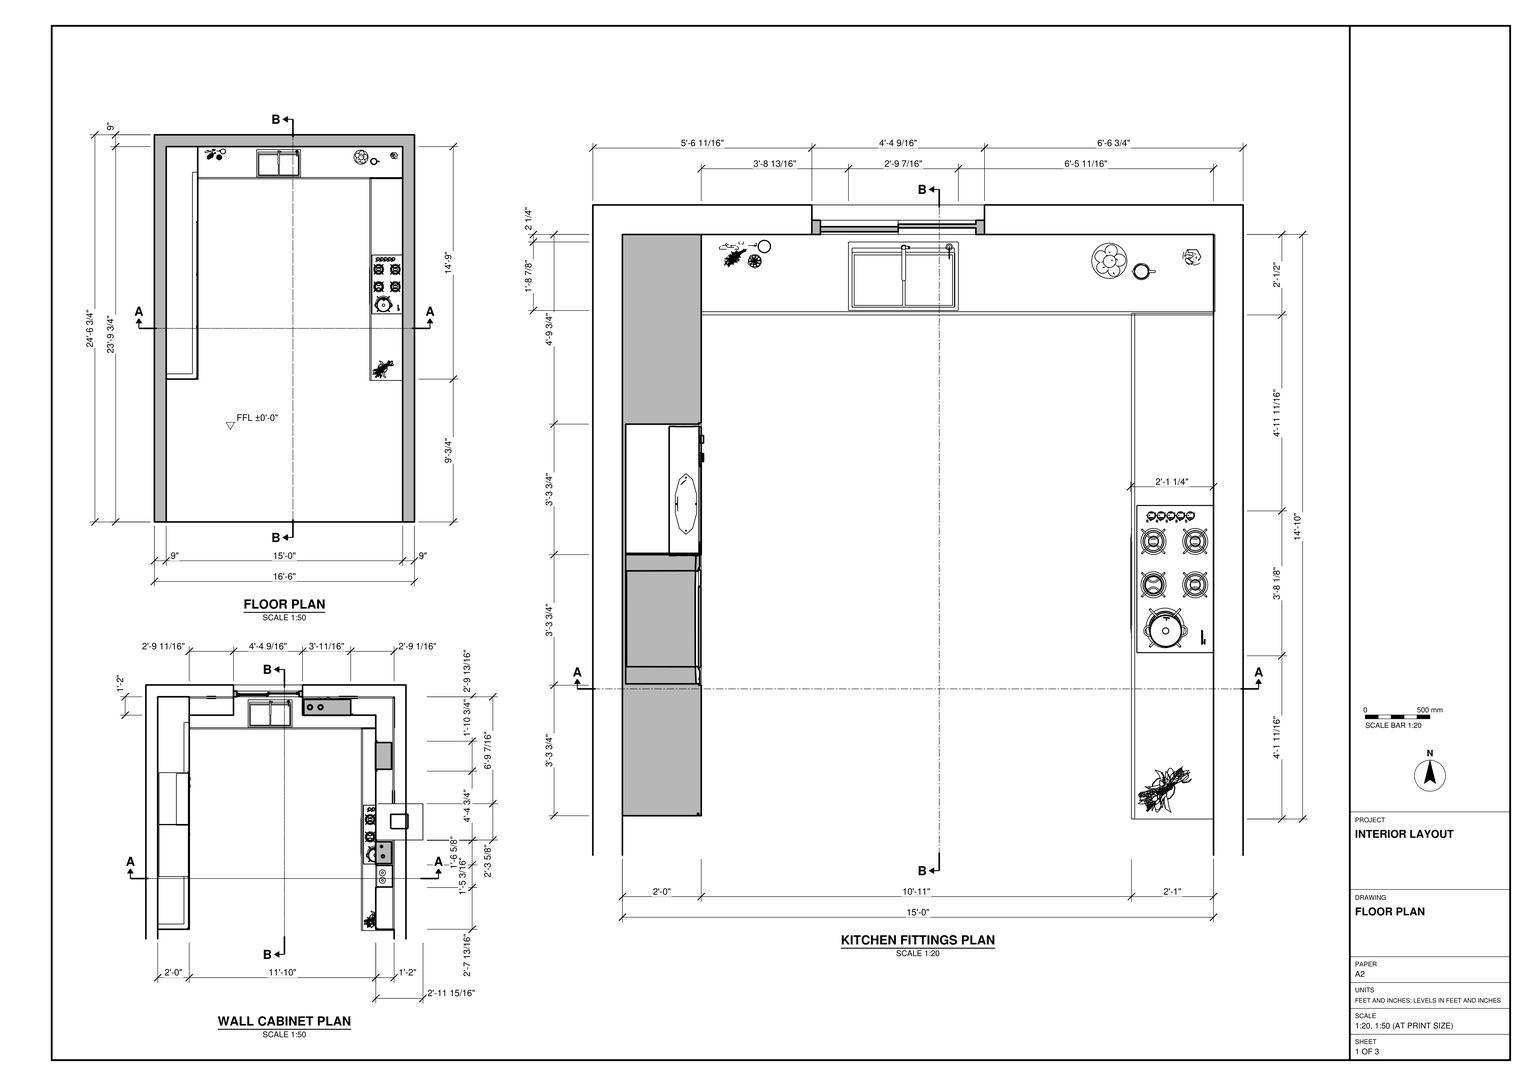
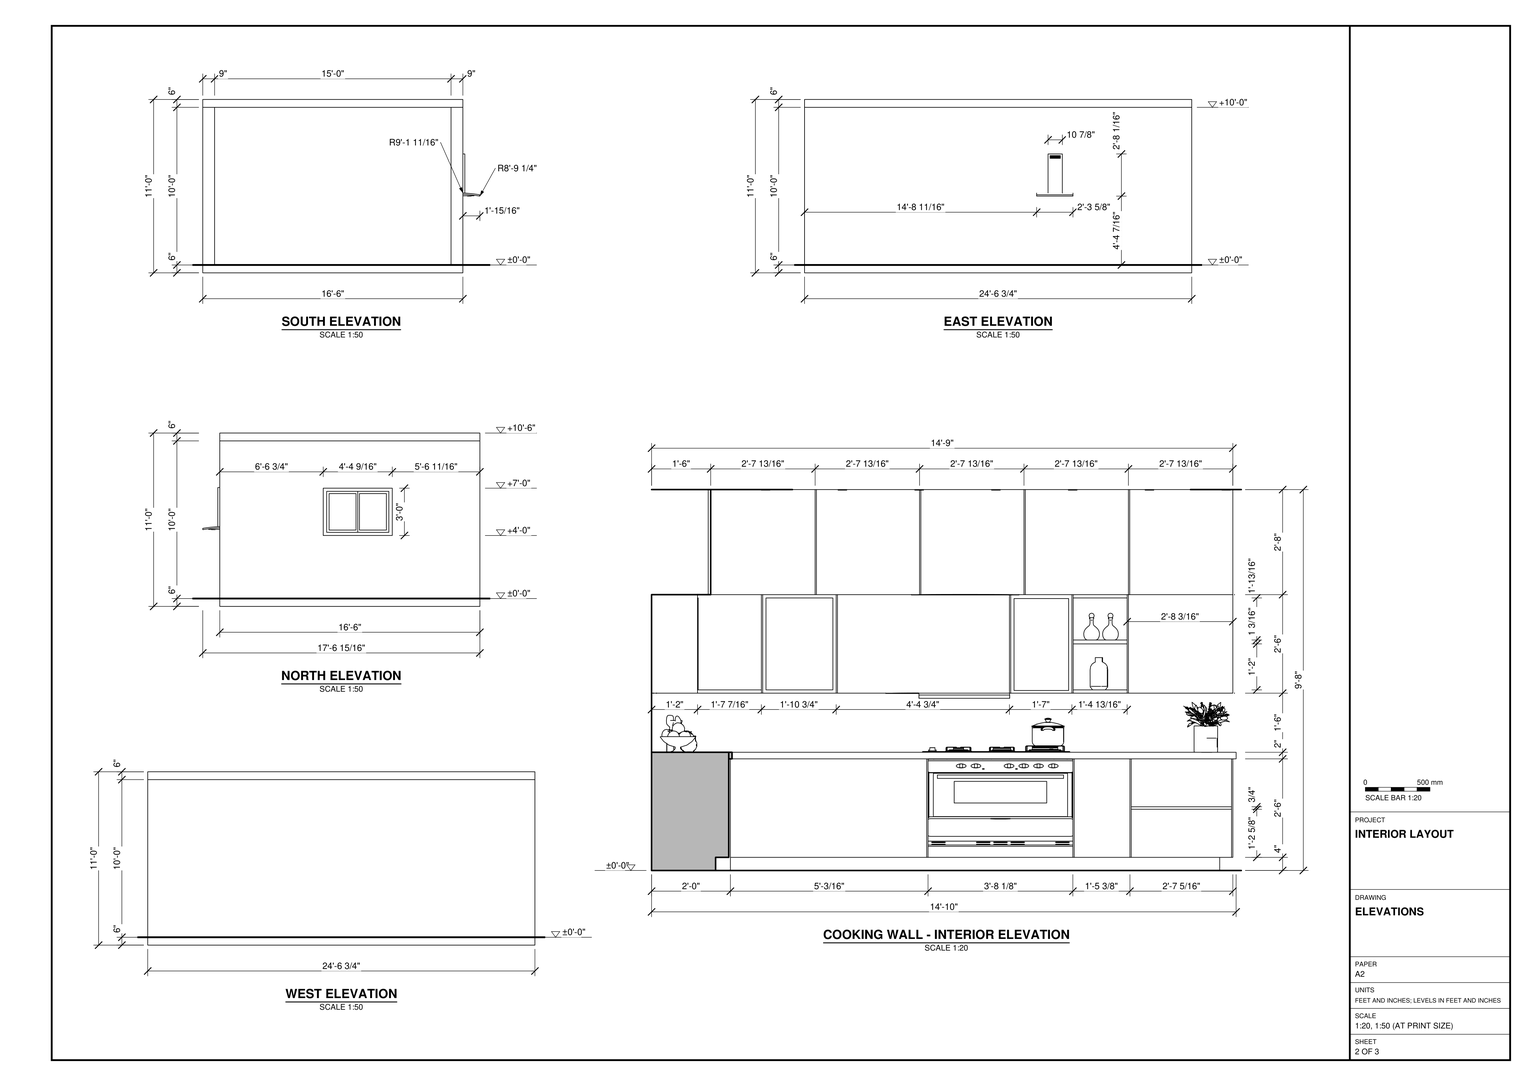
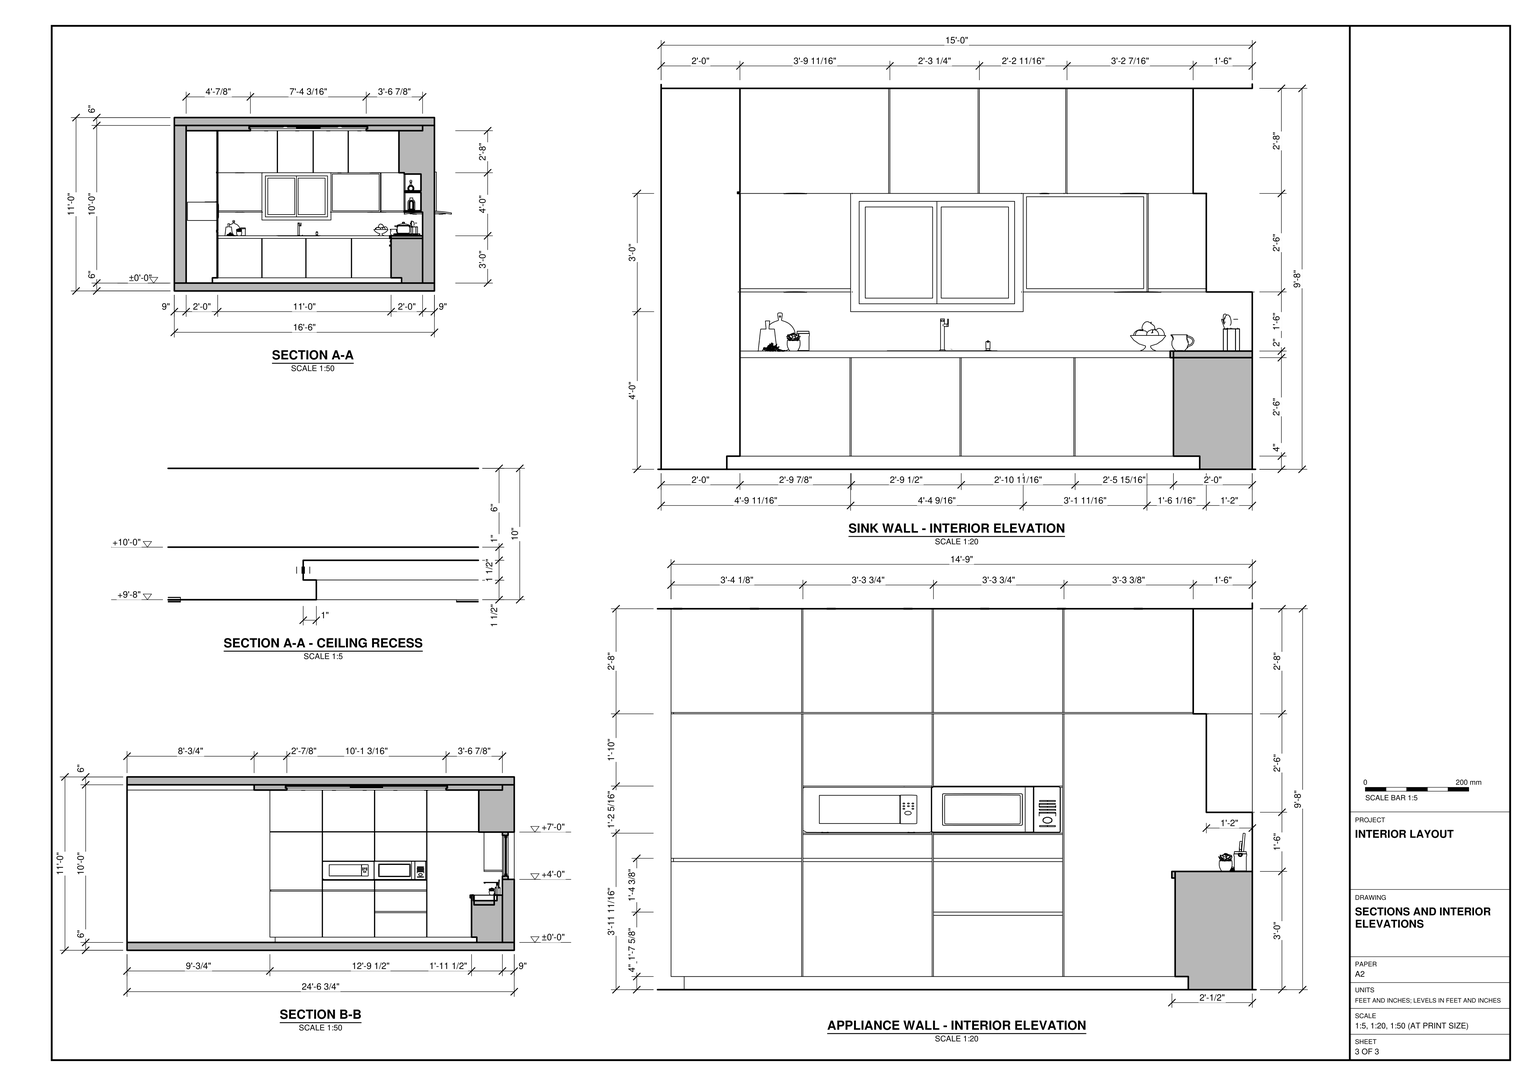
Build the kitchen interior in SketchUp from task_files/diagram_01.pdf. Work in feet and inches, with the finished floor at ±0'-0". The overall model extents, including the projection at the cooking wall, are 17'-6 15/16" wide, 24'-6 3/4" deep and 11'-0" high. Keep the room itself 15'-0" wide between the inside faces of the side walls. Model the 9" walls, the open south end, the floor and ceiling slabs, and the stepped ceiling recess shown in section.

Use the fittings plan to lay out the three cabinet runs and the interior elevations to divide their fronts. On the north wall, place the double-bowl sink and tap beneath the two-panel window, with base cupboards below the counter and wall cabinets around the opening. On the east wall, align the cooktop, oven and hood, and include the open shelf bay beside the hood. On the opposite wall, fit the two appliances side by side within the tall cabinetry. Leave the aisle and the floor toward the open end clear. Appliances, plants and loose countertop items may be any suitable library components placed as shown.

Keep the shell elements and each joinery piece in separate groups or components, and use components for repeated parts. Save one SketchUp model as output_files/u_shaped_kitchen_with_fitted_cabinetry.skp.

# SketchUp Ruby script. Lengths in inches.
U = 1.inch
M = Sketchup.active_model
def pt(a) = Geom::Point3d.new(a.map { |v| v * U })
def face(e, loops, mat)
  f = e.add_face(loops[0].map { |a| pt(a) })
  loops[1..].each { |l| e.add_face(l.map { |a| pt(a) }).erase! }
  f.material = f.back_material = mat if mat
  f
end
# faces: each face lists its corners as indices into pts; further lists are holes
def faces(e, pts, list, mat = nil) = list.each { |f| face(e, (f[0].is_a?(Array) ? f : [f]).map { |l| l.map { |i| pts[i] } }, mat) }
# xy, xz, yz: faces in a plane at the given z, y or x. An outline is a flat list of corners, or four numbers for a rectangle; further outlines are holes
def ring(l) = l.size == 4 ? [[l[0], l[1]], [l[2], l[1]], [l[2], l[3]], [l[0], l[3]]] : l.each_slice(2).to_a
def flat(e, list, mat, &to3) = list.each { |f| face(e, (f[0].is_a?(Array) ? f : [f]).map { |l| ring(l).map { |u, v| to3.(u, v) } }, mat) }
def xy(e, z, list, mat = nil) = flat(e, list, mat) { |x, y| [x, y, z] }
def xz(e, y, list, mat = nil) = flat(e, list, mat) { |x, z| [x, y, z] }
def yz(e, x, list, mat = nil) = flat(e, list, mat) { |y, z| [x, y, z] }
def lines(e, pts, list) = list.each { |a, b| e.add_line(pt(pts[a]), pt(pts[b])) }
# prism: a flat outline (further loops are holes) pulled along v
def prism(e, loops, v, mat = nil)
  f = face(e, loops, mat); d = Geom::Vector3d.new(v.map { |x| x * U })
  f.pushpull(f.normal.samedirection?(d) ? d.length : -d.length)
end
def box(e, o, s, mat = nil) = prism(e, [[o, [o[0] + s[0], o[1], o[2]], [o[0] + s[0], o[1] + s[1], o[2]], [o[0], o[1] + s[1], o[2]]]], [0, 0, s[2]], mat)
def at(x, y, z, deg = 0) = Geom::Transformation.translation(pt([x, y, z])) * Geom::Transformation.rotation(ORIGIN, Z_AXIS, deg.degrees)
def axes(o, x, y, z) = Geom::Transformation.new([*x, 0, *y, 0, *z, 0, *pt(o).to_a, 1])
def part(name) = M.definitions.add(name)
# library, detail: a bought-in or finely detailed component or shape, given as its bounding box
def library(name, o, s) = part(name).tap { |d| box(d.entities, o, s) }
def detail(e, o, s) = box(e.add_group.entities, o, s)
def put(e, d, t, mat = nil) = e.add_instance(d, t).tap { |i| i.material = mat if mat }
def group(e, t, mat = nil) = e.add_group.tap { |g| g.transformation = t; g.material = mat if mat }.entities
root = M.entities
M.materials.add("0209 AP 9428 SKY PINK").color = [243, 236, 233]
M.materials.add("Emissive").color = [244, 243, 201]
M.materials.add("Generic").color = [193, 202, 184]
M.materials.add("Glass Thin Clear 001\#1").color = [29, 27, 27]
M.materials["Glass Thin Clear 001\#1"].alpha = 0.1
M.materials.add("Granite Black Pearl 150cm").color = [48, 48, 48]
M.materials.add("Tiles Simple 02 100cm\#1").color = [183, 183, 183]
M.materials.add("[Color M08]").color = [30, 30, 30]
M.materials.add("[Translucent_Glass_Safety]").color = [204, 235, 244]
M.materials["[Translucent_Glass_Safety]"].alpha = 0.5
M.materials.add("[Translucent_Glass_Sky_Reflection]").color = [125, 138, 183]
M.materials["[Translucent_Glass_Sky_Reflection]"].alpha = 0.52
M.materials.add("[Wood Floor Light]").color = [204, 176, 127]
c1 = library("Microwave 116-15",[-11.91,-6.3,0],[23.82,12.61,15.33])
c2 = library("Microwave 116-11",[-7.27,-5.23,0],[14.54,10.46,7.87])
c3 = library("Utensils",[0,-0.54,-0.24],[6.34,6.28,13.37])
c4 = library("Glass_Apothecary_Jar",[-11.5,-3.52,0],[30.82,7.02,10])
c5 = library("ACCESS \#103",[-1.07,0,-1.17],[14.88,24.44,20.18])
c6 = library("Kitchen Utensils - Pot",[14.77,-5.37,0.11],[13.29,9.84,8.54])
c7 = library("kitchen utensils1",[32.53,200.33,5.92],[41.29,12.2,17.07])
c8 = part("Sliding window")
xy(c8.entities,0,[[0,0,4.33,55.51]])
xy(c8.entities,2.76,[[0,2.76,2,27.76],[3.15,2.76,4.33,27.76],[0,27.76,0.82,52.76],[0.82,27.76,2.36,52.76],[2.36,27.76,4.33,52.76]])
xy(c8.entities,4.72,[[2,4.72,2.4,26.38],[2.76,4.72,3.15,26.38],[0.82,29.13,1.22,50.79],[1.97,29.13,2.36,50.79]])
xy(c8.entities,36.61,[[2,4.72,2.4,26.38],[2.76,4.72,3.15,26.38],[0.82,29.13,1.22,50.79],[1.97,29.13,2.36,50.79]])
xy(c8.entities,38.58,[[0,2.76,2,27.76],[3.15,2.76,4.33,27.76],[0,27.76,0.82,52.76],[0.82,27.76,2.36,52.76],[2.36,27.76,4.33,52.76]])
xy(c8.entities,41.34,[[0,0,4.33,55.51]])
xz(c8.entities,0,[[0,0,4.33,41.34]])
xz(c8.entities,2.76,[[0,2.76,2,38.58],[3.15,2.76,4.33,38.58]])
xz(c8.entities,4.72,[[2,4.72,2.4,36.61],[2.76,4.72,3.15,36.61]])
xz(c8.entities,26.38,[[2,4.72,2.4,36.61],[2.76,4.72,3.15,36.61]])
xz(c8.entities,27.76,[[0.82,2.76,2,38.58],[2,2.76,2.36,38.58],[2.36,2.76,3.15,38.58]])
xz(c8.entities,29.13,[[0.82,4.72,1.22,36.61],[1.97,4.72,2.36,36.61]])
xz(c8.entities,50.79,[[0.82,4.72,1.22,36.61],[1.97,4.72,2.36,36.61]])
xz(c8.entities,52.76,[[0,2.76,0.82,38.58],[0.82,2.76,2.36,38.58],[2.36,2.76,4.33,38.58]])
xz(c8.entities,55.51,[[0,0,4.33,41.34]])
yz(c8.entities,0,[[[0,0,55.51,41.34],[2.76,2.76,52.76,38.58]]])
yz(c8.entities,0.82,[[[27.76,2.76,52.76,38.58],[29.13,4.72,50.79,36.61]]])
yz(c8.entities,1.22,[[29.13,4.72,50.79,36.61]],"[Translucent_Glass_Sky_Reflection]")
yz(c8.entities,1.97,[[29.13,4.72,50.79,36.61]],"[Translucent_Glass_Sky_Reflection]")
yz(c8.entities,2,[[[2.76,2.76,27.76,38.58],[4.72,4.72,26.38,36.61]]])
yz(c8.entities,2.36,[[[27.76,2.76,52.76,38.58],[29.13,4.72,50.79,36.61]]])
yz(c8.entities,2.4,[[4.72,4.72,26.38,36.61]],"[Translucent_Glass_Safety]")
yz(c8.entities,2.76,[[4.72,4.72,26.38,36.61]],"[Translucent_Glass_Safety]")
yz(c8.entities,3.15,[[[2.76,2.76,27.76,38.58],[4.72,4.72,26.38,36.61]]])
yz(c8.entities,4.33,[[[0,0,55.51,41.34],[2.76,2.76,52.76,38.58]]])
c9 = library("PV977NSS_GEProfile",[-17.9375,-27.5625,-0.25],[35.95,27.64,32.08])
c10 = library("Cooktop+Brastemp+Ative!",[2.49,1.09,0.39],[33.46,18.11,1.98])
c11 = library("PointStove",[0,-0.4,0],[23.23,24.97,35.55])
c12 = library("Apple 73-11",[-5.39,-5.39,0],[10.78,10.78,8.98])
c13 = library("Vase 193 003",[-7.6875,-7.21,0],[16.1875,14.01,15.28])
c14 = library("Jug 155 004",[-2.86,-2.52,0],[7.11,5.04,4.97])
c15 = library("Bathroom Fixture 02 22-64",[-3.05,-2.36,0],[6.1,4.72,3.64])
c16 = library("Bottle 01 97-27",[-2.41,-2.41,0],[4.82,4.82,8.18])
c17 = library("Bottle 03 97-27",[-1.45,-1.45,0],[2.9,2.9,11.4])
c18 = library("Vase 010",[-2.69,-2.69,0.01],[5.38,5.38,9.84])
c19 = library("white sink",[101.38,33.55,27.24],[20.87,33.46,17.21])
c20 = library("Tlon Light 650 Ceiling 152 007",[-12.8,-12.8,-3.78],[25.6,25.6,3.58])
c21 = library("Group\#25",[-0.5,-0.5,-0.1],[2,177,0.2])
c22 = library("Group\#26",[-0.5,-0.5,-0.1],[70.75,2,0.2])
c23 = library("Group\#27",[-0.5,-0.5,-0.1],[34.6875,2,0.2])
c24 = library("Group\#28",[-0.5,-0.5,-0.1],[34.6875,2,0.2])
c25 = library("Group\#30",[-0.5,-0.5,-0.1],[2.75,164,0.2])
c26 = library("Group\#29",[-0.5,-0.5,-0.1],[42.8125,2.75,0.2])
c27 = library("Group\#31",[-0.5,-0.5,-0.1],[13.9375,2,0.2])
c28 = library("Group\#32",[-0.5,-0.5,0],[90.2,1,1.5])
c29 = library("Group\#33",[-0.5,-0.5,0],[1,123.2,1.5])
c30 = library("Group\#34",[-0.5,-0.5,0],[91.2,1,1.5])
c31 = library("Group\#35",[-0.5,-0.5,0],[1,124.2,1.5])
c32 = library("Group\#36",[-0.5,-0.5,-0.1],[4.4375,102.5625,0.2])
c33 = library("Group\#37",[-0.5,-0.5,-0.1],[4.4375,102.5625,0.2])
xy(root,-6,[[0,0,198,294.75]])
xy(root,0,[[0,0,9,0,9,285.75,189.4375,285.75,189.4375,262.25,189,262.25,189,0,198,0,198,294.75,0,294.75],[9,112.75,9,285.75,33,285.75,33,266.25,29,266.25,29,112.75],[173,112.75,189,261.75],[189,262.25,189.4375,285.75],[33,266.25,189,285.75]])
xy(root,0,[[9,0,189,0,189,112.75,173,112.75,173,261.75,189,261.75,189,266.25,29,266.25,29,112.75,9,112.75]],"Tiles Simple 02 100cm\#1")
xy(root,4,[[9,108.75,9,112.75,29,112.75,29,266.25,33,266.25,33,228.4,32.25,228.4,32.25,228,33,228,33,188.65,32.25,188.65,32.25,188.25,33,188.25,33,148.9,32.25,148.9,32.25,148.5,33,148.5,33,108.75,32.25,108.75,32.25,109.5,31.85,109.5,31.85,108.75],[165.75,108.75,165.75,109.15,165,109.15,165,139.6875,165.75,139.6875,165.75,140.09,165,140.09,165,157.0625,165.75,157.0625,165.75,157.46,165,157.46,165,201.5625,165.75,201.5625,165.75,201.96,165,201.96,165,261.75,173,261.75,173,112.75,169,112.75,169,108.75],[169,108.75,189,112.75],[33,262.25,33,266.25,189,266.25,189,262.25,135.0625,262.25,135.0625,263,134.66,263,134.66,262.25,100.375,262.25,100.375,263,99.98,263,99.98,262.25,66.89,262.25,66.89,263,66.49,263,66.49,262.25]])
xy(root,7.75,[[165,157.46,188,201.5625]])
xy(root,18.65,[[165,109.15,165.75,139.6875]],"[Color M08]")
xy(root,19.4,[[165,109.15,165.75,139.6875]],"[Color M08]")
xy(root,22.625,[[32.25,188.65,33,228]],"[Color M08]")
xy(root,23.625,[[32.25,188.65,33,228]],"[Color M08]")
xy(root,31.8125,[[78.93,263.61,110.08,281.61]],"[Color M08]")
xy(root,34,[[165.75,108.75,165.75,109.15,165,109.15,165,139.6875,165.75,139.6875,165.75,140.09,165,140.09,165,157.0625,165.75,157.0625,165.75,157.46,188,157.46,188,201.5625,165.75,201.5625,165.75,201.96,165,201.96,165,261.25,189,261.25,189,108.75],[165,261.25,189,261.75],[66.49,262.25,66.89,263],[99.98,262.25,100.375,263],[134.66,262.25,135.0625,263]])
xy(root,34,[[164,107.75,165,261.25],[165,107.75,189,108.75],[165,108.75,165.75,109.15],[33,261.25,33,262.25,189,262.25,189,261.75,164,261.75,164,261.25],[164,261.25,165,261.75]],"Granite Black Pearl 150cm")
xy(root,34,[[165,139.6875,165.75,140.09],[165,157.0625,165.75,157.46],[165,157.46,188,201.5625],[165,201.5625,165.75,201.96]],"[Color M08]")
xy(root,36,[[164,261.25,165,261.75],[165,261.25,189,261.75]])
xy(root,36,[[164,107.75,165,261.25],[165,107.75,189,261.25],[33,261.25,164,261.25,164,261.75,189,261.75,189,262.25,33,262.25],[[33,262.25,189,285.75],[78.93,263.61,110.08,281.61]]],"Granite Black Pearl 150cm")
xy(root,39,[[32.25,108.75,33,148.5],[32.25,148.9,33,188.25],[32.25,188.65,33,228]],"[Color M08]")
xy(root,40,[[32.25,108.75,33,148.5],[32.25,148.9,33,188.25],[32.25,188.65,33,228]],"[Color M08]")
xy(root,47.26,[[32.25,148.9,33,188.25],[32.25,188.65,33,228]],"[Color M08]")
xy(root,47.66,[[10,148.9,32.25,188.25],[10,188.65,32.25,228]],"[Color M08]")
xy(root,48,[[66.6875,285.75,119.25,294.75]])
xy(root,54,[[175,108.75,175,140.54,175.75,140.54,175.75,140.9375,175,140.9375,175,157.35,175.75,157.35,175.75,157.75,175,157.75,175,176.38,175.75,176.38,175.75,176.78,175,176.78,175,229.14,175.75,229.14,175.75,229.54,175,229.54,175,251.91,175.75,251.91,175.75,252.3125,175,252.3125,175,271.75,157.34,271.75,157.34,272.5,156.9375,272.5,156.9375,271.75,119.25,271.75,119.25,284.75,188,284.75,188,108.75,176.15,108.75,176.15,109.5,175.75,109.5,175.75,108.75],[33,271.75,66.6875,284.75]],"Generic")
xy(root,54.8125,[[174.8,158.75,175,175.38]])
xy(root,55,[[174.8,230.54,175,250.91],[120.25,271.55,155.9375,271.75]])
xy(root,55,[[175,140.9375,187.75,157.35],[175,230.54,187,250.91],[120.25,271.75,155.9375,283.75]],"[Wood Floor Light]")
xy(root,61.6,[[10,148.9,32.25,188.25]])
xy(root,61.6,[[10,188.65,32.25,228]],"[Color M08]")
xy(root,62,[[32.25,148.9,33,188.25],[32.25,188.65,33,228]],"[Color M08]")
xy(root,68.29,[[186,158.75,187,175.38],[186,230.54,187,250.91]],"Emissive")
xy(root,68.29,[[175.2,158.75,186,175.38],[175.2,230.54,186,250.91]],"[Wood Floor Light]")
xy(root,69,[[120.25,282.75,155.9375,283.75]],"Emissive")
xy(root,69,[[175.75,140.9375,187.75,157.35],[175.2,158.75,187,175.38],[175.2,230.54,187,250.91],[120.25,271.95,155.9375,282.75]],"[Wood Floor Light]")
xy(root,70.17,[[120.25,271.95,155.9375,283.75]],"[Wood Floor Light]")
xy(root,70.1875,[[175.75,140.9375,187.75,157.35]],"[Wood Floor Light]")
xy(root,82.8125,[[174.8,158.75,175,175.38]])
xy(root,83,[[174.8,230.54,175,250.91],[120.25,271.55,132.1875,271.75],[132.1875,271.55,155.9375,271.75]])
xy(root,83,[[186,158.75,187,175.38],[186,230.54,187,250.91],[132.1875,282.75,155.9375,283.75]],"Emissive")
xy(root,83,[[175,140.9375,187.75,157.35],[175,230.54,186,250.91],[120.25,271.75,132.1875,282.75],[132.1875,271.75,155.9375,282.75],[120.25,282.75,132.1875,283.75]],"[Wood Floor Light]")
xy(root,84,[[175.75,108.75,176.15,109.5],[66.6875,285.75,119.25,294.75]])
xy(root,84,[[171,108.75,171,140.15,171.75,140.15,171.75,140.55,171,140.55,171,171.95,171.75,171.95,171.75,172.35,171,172.35,171,203.75,171.75,203.75,171.75,204.15,171,204.15,171,235.55,171.75,235.55,171.75,235.95,171,235.95,171,267.75,132.59,267.75,132.59,268.5,132.1875,268.5,132.1875,270.75,174,270.75,174,108.75,172.15,108.75,172.15,109.5,171.75,109.5,171.75,108.75],[33,267.75,33,270.75,66.6875,270.75,66.6875,271.75,79.625,271.75,79.625,267.75,78.66,267.75,78.66,268.5,78.26,268.5,78.26,267.75],[79.625,267.75,79.625,271.75,66.6875,271.75,66.6875,285.75,119.25,285.75,119.25,270.75,132.1875,270.75,132.1875,267.75,105.91,267.75,105.91,268.5,105.51,268.5,105.51,267.75]],"Generic")
xy(root,84,[[32.25,108.75,33,148.5],[32.25,148.9,33,188.25],[32.25,188.65,33,228],[32.25,228.4,33,267.75]],"[Color M08]")
xy(root,84.4,[[32.25,108.75,33,148.5],[32.25,148.9,33,188.25],[32.25,188.65,33,228],[32.25,228.4,33,267.75]],"[Color M08]")
xy(root,116,[[9,96.75,9,108.75,31.85,108.75,31.85,109.5,32.25,109.5,32.25,108.75,33,108.75,33,96.75],[32.25,148.5,33,148.9],[32.25,188.25,33,188.65],[32.25,228,33,228.4]])
xy(root,116,[[[33,96.75,33,267.75,78.26,267.75,78.26,268.5,78.66,268.5,78.66,267.75,105.51,267.75,105.51,268.5,105.91,268.5,105.91,267.75,132.1875,267.75,132.1875,268.5,132.59,268.5,132.59,267.75,171,267.75,171,235.95,171.75,235.95,171.75,235.55,171,235.55,171,204.15,171.75,204.15,171.75,203.75,171,203.75,171,172.35,171.75,172.35,171.75,171.95,171,171.95,171,140.55,171.75,140.55,171.75,140.15,171,140.15,171,108.75,171.75,108.75,171.75,109.5,172.15,109.5,172.15,108.75,189,108.75,189,96.75],[57.9,121.65,146.1,242.85]]],"0209 AP 9428 SKY PINK")
xy(root,116,[[9,108.75,31.85,108.75,31.85,109.5,32.25,109.5,32.25,108.75,33,108.75,33,148.5,32.25,148.5,32.25,148.9,33,148.9,33,188.25,32.25,188.25,32.25,188.65,33,188.65,33,228,32.25,228,32.25,228.4,33,228.4,33,285.75,9,285.75],[171,108.75,171,140.15,171.75,140.15,171.75,140.55,171,140.55,171,171.95,171.75,171.95,171.75,172.35,171,172.35,171,203.75,171.75,203.75,171.75,204.15,171,204.15,171,235.55,171.75,235.55,171.75,235.95,171,235.95,171,267.75,132.59,267.75,132.59,268.5,132.1875,268.5,132.1875,267.75,105.91,267.75,105.91,268.5,105.51,268.5,105.51,267.75,78.66,267.75,78.66,268.5,78.26,268.5,78.26,267.75,33,267.75,33,285.75,189,285.75,189,108.75,172.15,108.75,172.15,109.5,171.75,109.5,171.75,108.75]],"Generic")
xy(root,117.5,[[56.9,120.65,147.1,121.65],[56.9,121.65,57.9,242.85],[146.1,121.65,147.1,243.85],[56.9,242.85,146.1,243.85]],"0209 AP 9428 SKY PINK")
xy(root,119,[[[56.9,120.65,147.1,243.85],[82.74,132.49,86.18,234.05],[124.3,132.49,127.74,234.05]]],"0209 AP 9428 SKY PINK")
xy(root,120,[[0,0,0,294.75,198,294.75,198,0,189,0,189,285.75,9,285.75,9,0],[9,0,189,96.75],[9,96.75,189,285.75]])
xy(root,126,[[0,0,198,294.75]])
xz(root,0,[[0,-6,198,0],[0,0,9,120],[9,0,189,120],[189,0,198,120],[0,120,198,126]])
xz(root,96.75,[[9,116,189,120]])
xz(root,107.75,[[164,34,165,36],[165,34,189,36]],"Granite Black Pearl 150cm")
xz(root,108.75,[[9,4,31.85,116],[32.25,4,33,39],[165.75,4,189,34],[32.25,40,33,84],[175,54,175.75,84],
  [176.15,54,189,84],[171,84,171.75,116],[172.15,84,189,116],[32.25,84.4,33,116]],"Generic")
xz(root,109.15,[[165,4,165.75,18.65],[165,19.4,165.75,34]],"Generic")
xz(root,109.5,[[175.75,54,176.15,84]])
xz(root,109.5,[[31.85,4,32.25,116],[171.75,84,172.15,116]],"[Color M08]")
xz(root,112.75,[[9,0,29,4],[173,0,189,4]],"[Color M08]")
xz(root,120.65,[[56.9,117.5,57.9,119]],"0209 AP 9428 SKY PINK")
xz(root,121.65,[[57.9,116,146.1,117.5]],"0209 AP 9428 SKY PINK")
xz(root,132.49,[[82.74,119,86.18,119.9],[124.3,119,127.74,119.9]],"0209 AP 9428 SKY PINK")
xz(root,139.6875,[[165,4,165.75,18.65],[165,19.4,165.75,34]],"[Color M08]")
xz(root,140.09,[[165,4,165.75,34]],"[Color M08]")
xz(root,140.15,[[171,84,171.75,116]],"[Color M08]")
xz(root,140.54,[[175,54,175.75,84]],"[Color M08]")
xz(root,140.55,[[171,84,171.75,116]],"[Color M08]")
xz(root,140.9375,[[175,54,175.75,55]])
xz(root,140.9375,[[175.75,55,187.75,69],[175.75,70.1875,187.75,83],[175,83,175.75,84]],"[Wood Floor Light]")
xz(root,148.5,[[32.25,4,33,39],[32.25,40,33,84],[32.25,84.4,33,116]],"[Color M08]")
xz(root,148.9,[[32.25,4,33,39],[32.25,40,33,47.26],[10,47.66,32.25,61.6],[32.25,62,33,84],[32.25,84.4,33,116]],"[Color M08]")
xz(root,157.0625,[[165,4,165.75,34]],"[Color M08]")
xz(root,157.35,[[175,54,175.75,55],[175,83,175.75,84]])
xz(root,157.35,[[175.75,55,187.75,69],[175.75,70.1875,187.75,83]],"[Wood Floor Light]")
xz(root,157.46,[[165,4,165.75,7.35],[165,7.35,165.75,7.75]])
xz(root,157.46,[[165.75,7.75,188,34]],"[Color M08]")
xz(root,157.75,[[175,54,175.75,84]],"[Color M08]")
xz(root,158.75,[[174.8,54.8125,175,82.8125]])
xz(root,158.75,[[175,54.8125,175,68.1,175.2,68.29,187,68.29,187,55],[175,68.1,175,68.8125,175.2,69,175.2,68.29],[175,68.8125,175,82.8125,186,83,187,83,187,69,175.2,69]],"[Wood Floor Light]")
xz(root,171.95,[[171,84,171.75,116]],"[Color M08]")
xz(root,172.35,[[171,84,171.75,116]],"[Color M08]")
xz(root,175.38,[[174.8,54.8125,175,82.8125]])
xz(root,175.38,[[175,54.8125,187,55,187,68.29,175.2,68.29,175,68.1],[175,68.1,175.2,68.29,175.2,69,175,68.8125],[175,68.8125,175.2,69,187,69,187,83,186,83,175,82.8125]],"[Wood Floor Light]")
xz(root,176.38,[[175,54,175.75,84]],"[Color M08]")
xz(root,176.78,[[175,54,175.75,84]],"[Color M08]")
xz(root,188.25,[[32.25,4,33,39],[32.25,40,33,47.26],[10,47.66,32.25,61.6],[32.25,62,33,84],[32.25,84.4,33,116]],"[Color M08]")
xz(root,188.65,[[10,47.66,32.25,61.6]])
xz(root,188.65,[[32.25,4,33,22.625],[32.25,23.625,33,39],[32.25,40,33,47.26],[32.25,62,33,84],[32.25,84.4,33,116]],"[Color M08]")
xz(root,201.5625,[[165,4,165.75,7.35],[165,7.35,165.75,7.75]])
xz(root,201.5625,[[165.75,7.75,188,34]],"[Color M08]")
xz(root,201.96,[[165,4,165.75,34]],"[Color M08]")
xz(root,203.75,[[171,84,171.75,116]],"[Color M08]")
xz(root,204.15,[[171,84,171.75,116]],"[Color M08]")
xz(root,228,[[32.25,4,33,22.625],[32.25,23.625,33,39],[32.25,40,33,47.26],[32.25,62,33,84]])
xz(root,228,[[10,47.66,32.25,61.6],[32.25,84.4,33,116]],"[Color M08]")
xz(root,228.4,[[32.25,4,33,84],[32.25,84.4,33,116]],"[Color M08]")
xz(root,229.14,[[175,54,175.75,84]],"[Color M08]")
xz(root,229.54,[[175,54,175.75,84]],"[Color M08]")
xz(root,230.54,[[174.8,55,175,83]])
xz(root,230.54,[[175,55,187,68.29],[175,68.29,175.2,69],[175,69,187,83]],"[Wood Floor Light]")
xz(root,234.05,[[82.74,119,86.18,119.9],[124.3,119,127.74,119.9]],"0209 AP 9428 SKY PINK")
xz(root,235.55,[[171,84,171.75,116]],"[Color M08]")
xz(root,235.95,[[171,84,171.75,116]],"[Color M08]")
xz(root,242.85,[[57.9,116,146.1,117.5]],"0209 AP 9428 SKY PINK")
xz(root,250.91,[[174.8,55,175,83]])
xz(root,250.91,[[175,55,187,68.29],[175,68.29,175.2,69],[175,69,187,83]],"[Wood Floor Light]")
xz(root,251.91,[[175,54,175.75,84]],"[Color M08]")
xz(root,252.3125,[[175,54,175.75,55],[175,55,175.75,84]],"[Color M08]")
xz(root,261.25,[[33,34,189,36]],"Granite Black Pearl 150cm")
xz(root,261.75,[[173,0,173,4,165,4,165,34,189,34,189,0],[164,34,165,36],[165,34,189,36]])
xz(root,262.25,[[33,34,189,36]])
xz(root,262.25,[[33,4,66.49,34],[66.89,4,99.98,34],[100.375,4,134.66,34],[135.0625,4,189,34]],"Generic")
xz(root,263,[[66.49,4,66.89,34],[99.98,4,100.375,34],[134.66,4,135.0625,34]],"[Color M08]")
xz(root,263.61,[[78.93,31.8125,110.08,36]])
xz(root,266.25,[[29,0,189,4]],"[Color M08]")
xz(root,267.75,[[32.25,84,33,84.4]])
xz(root,267.75,[[33,84,78.26,116],[78.66,84,105.51,116],[105.91,84,132.1875,116],[132.59,84,171,116]],"Generic")
xz(root,268.5,[[78.26,84,78.66,116],[105.51,84,105.91,116],[132.1875,84,132.59,116]],"[Color M08]")
xz(root,271.55,[[120.25,55,155.9375,83]],"Glass Thin Clear 001\#1")
xz(root,271.75,[[33,55,66.6875,84],[157.34,55,175,84]],"Generic")
xz(root,271.75,[[120.25,55,155.9375,83]],"Glass Thin Clear 001\#1")
xz(root,271.75,[[33,54,66.6875,55],[[119.25,54,156.9375,84],[120.25,55,155.9375,83]],[157.34,54,175,55]],"[Color M08]")
xz(root,271.95,[[120.25,69,155.9375,70.17]],"[Wood Floor Light]")
xz(root,272.5,[[156.9375,54,157.34,84]],"[Color M08]")
xz(root,281.61,[[78.93,31.8125,110.08,36]])
xz(root,283.75,[[120.25,55,155.9375,69],[120.25,70.17,155.9375,83]],"[Wood Floor Light]")
xz(root,285.75,[[9,0,33,116],[33,0,189,31.8125],[33,31.8125,189,36],[9,116,189,120]])
xz(root,285.75,[[33,36,189,36,189,54,119.25,54,119.25,48,66.6875,48,66.6875,54,33,54]],"0209 AP 9428 SKY PINK")
xz(root,294.75,[[0,-6,198,0],[[0,0,198,120],[66.6875,48,119.25,84]],[0,120,198,126]])
yz(root,0,[[0,-6,294.75,0],[0,0,294.75,120],[0,120,294.75,126]])
yz(root,9,[[0,0,112.75,0,112.75,4,108.75,4,108.75,116,0,116],[0,116,96.75,120],[96.75,116,285.75,120]])
yz(root,9,[[112.75,0,285.75,0,285.75,116,108.75,116,108.75,4,112.75,4]],"[Color M08]")
yz(root,10,[[148.9,47.66,188.25,61.6],[188.65,47.66,228,61.6]])
yz(root,29,[[112.75,0,266.25,4]],"[Color M08]")
yz(root,31.85,[[108.75,84,109.5,84.4],[108.75,84.4,109.5,116]])
yz(root,31.85,[[108.75,4,109.5,39],[108.75,39,109.5,40],[108.75,40,109.5,84]],"[Color M08]")
yz(root,32.25,[[108.75,4,109.5,39],[148.5,4,148.9,84],[188.25,4,188.65,84],[228,4,228.4,84],[188.65,22.625,228,23.625],
  [108.75,39,109.5,40],[148.9,39,188.25,40],[188.65,39,228,40],[108.75,40,109.5,84],[148.9,47.26,188.25,47.66],
  [188.65,47.26,228,47.66],[148.9,61.6,188.25,62],[188.65,61.6,228,62],[108.75,84,109.5,84.4],[108.75,84.4,109.5,116],
  [148.5,84.4,148.9,116],[188.25,84.4,188.65,116],[228,84.4,228.4,116]],"[Color M08]")
yz(root,33,[[262.25,31.8125,267.75,36],[267.75,31.8125,285.75,36],[261.25,34,262.25,36],[271.75,54,285.75,84],[267.75,84,285.75,116]])
yz(root,33,[[108.75,4,148.5,39],[148.9,4,188.25,39],[188.65,4,228,22.625],[228.4,4,262.25,4,262.25,34,261.25,34,261.25,36,285.75,36,285.75,54,271.75,54,271.75,84,228.4,84],[188.65,23.625,228,39],
  [108.75,40,148.5,84],[148.9,40,188.25,47.26],[188.65,40,228,47.26],[148.9,62,188.25,84],[188.65,62,228,84],
  [108.75,84.4,148.5,116],[148.9,84.4,188.25,116],[188.65,84.4,228,116],[228.4,84.4,267.75,116]],"Generic")
yz(root,57.9,[[121.65,116,242.85,117.5]],"0209 AP 9428 SKY PINK")
yz(root,66.49,[[262.25,4,263,34]],"[Color M08]")
yz(root,66.6875,[[285.75,48,294.75,84]])
yz(root,66.6875,[[271.75,55,285.75,84]],"Generic")
yz(root,66.6875,[[271.75,54,285.75,55]],"[Color M08]")
yz(root,66.89,[[262.25,4,263,34]],"[Color M08]")
yz(root,78.26,[[267.75,84,268.5,116]],"[Color M08]")
yz(root,78.66,[[267.75,84,268.5,116]],"[Color M08]")
yz(root,78.93,[[263.61,31.8125,281.61,36]])
yz(root,82.74,[[132.49,119,234.05,119.9]],"0209 AP 9428 SKY PINK")
yz(root,86.18,[[132.49,119,234.05,119.9]],"0209 AP 9428 SKY PINK")
yz(root,99.98,[[262.25,4,263,34]],"[Color M08]")
yz(root,100.375,[[262.25,4,263,34]],"[Color M08]")
yz(root,105.51,[[267.75,84,268.5,116]],"[Color M08]")
yz(root,105.91,[[267.75,84,268.5,116]],"[Color M08]")
yz(root,110.08,[[263.61,31.8125,281.61,36]])
yz(root,119.25,[[285.75,48,285.75,54,271.75,54,271.75,84,294.75,84,294.75,48]],"Generic")
yz(root,120.25,[[271.55,55,271.75,83]])
yz(root,120.25,[[271.75,55,283.75,69],[271.75,69,271.95,70.17],[271.75,70.17,283.75,83]],"[Wood Floor Light]")
yz(root,124.3,[[132.49,119,234.05,119.9]],"0209 AP 9428 SKY PINK")
yz(root,127.74,[[132.49,119,234.05,119.9]],"0209 AP 9428 SKY PINK")
yz(root,132.1875,[[267.75,84,268.5,116]],"[Color M08]")
yz(root,132.59,[[267.75,84,268.5,116]],"[Color M08]")
yz(root,134.66,[[262.25,4,263,34]],"[Color M08]")
yz(root,135.0625,[[262.25,4,263,34]],"[Color M08]")
yz(root,146.1,[[121.65,116,242.85,117.5]],"0209 AP 9428 SKY PINK")
yz(root,147.1,[[242.85,117.5,243.85,119]],"0209 AP 9428 SKY PINK")
yz(root,155.9375,[[271.55,55,271.75,83]])
yz(root,155.9375,[[271.75,55,283.75,69],[271.75,69,271.95,70.17],[271.75,70.17,283.75,83]],"[Wood Floor Light]")
yz(root,156.9375,[[271.75,54,272.5,84]],"[Color M08]")
yz(root,157.34,[[271.75,54,272.5,55]])
yz(root,157.34,[[271.75,55,272.5,84]],"[Color M08]")
yz(root,164,[[107.75,34,261.75,36]],"Granite Black Pearl 150cm")
yz(root,165,[[157.46,4,201.5625,7.35],[157.46,7.35,201.5625,7.75],[107.75,34,261.75,36]])
yz(root,165,[[109.15,4,139.6875,18.65],[140.09,4,157.0625,34],[201.96,4,261.75,34],[109.15,19.4,139.6875,34]],"Generic")
yz(root,165.75,[[108.75,4,109.15,34],[139.6875,4,140.09,34],[157.0625,4,157.46,34],[201.5625,4,201.96,34],[109.15,18.65,139.6875,19.4]],"[Color M08]")
yz(root,171,[[108.75,84,140.15,116],[140.55,84,171.95,116],[172.35,84,203.75,116],[204.15,84,235.55,116],[235.95,84,267.75,116]],"Generic")
yz(root,171.75,[[108.75,84,109.5,116],[140.15,84,140.55,116],[171.95,84,172.35,116],[203.75,84,204.15,116],[235.55,84,235.95,116]],"[Color M08]")
yz(root,172.15,[[108.75,84,109.5,116]],"[Color M08]")
yz(root,173,[[112.75,0,261.75,4]],"[Color M08]")
yz(root,174.8,[[158.75,54.8125,175.38,82.8125],[230.54,55,250.91,83]],"Glass Thin Clear 001\#1")
yz(root,175,[[108.75,54,140.54,84],[176.78,54,229.14,84],[252.3125,55,271.75,84]],"Generic")
yz(root,175,[[158.75,54.8125,175.38,82.8125],[230.54,55,250.91,83]],"Glass Thin Clear 001\#1")
yz(root,175,[[[157.75,54,176.38,84],[158.75,54.8125,175.38,82.8125]],[[229.54,54,251.91,84],[230.54,55,250.91,83]],[252.3125,54,271.75,55]],"[Color M08]")
yz(root,175,[[140.9375,54,157.35,55],[140.9375,83,157.35,84]],"[Wood Floor Light]")
yz(root,175.2,[[158.75,68.29,175.38,69],[230.54,68.29,250.91,69]],"[Wood Floor Light]")
yz(root,175.75,[[108.75,54,109.5,84]])
yz(root,175.75,[[176.38,54,176.78,84],[229.14,54,229.54,84],[251.91,54,252.3125,84]],"[Color M08]")
yz(root,175.75,[[140.54,54,140.9375,84],[157.35,54,157.75,84],[140.9375,69,157.35,70.1875]],"[Wood Floor Light]")
yz(root,176.15,[[108.75,54,109.5,84]],"[Color M08]")
yz(root,187,[[158.75,55,175.38,68.29],[230.54,55,250.91,68.29],[158.75,69,175.38,83],[230.54,69,250.91,83]],"[Wood Floor Light]")
yz(root,187.75,[[140.9375,55,157.35,69],[140.9375,70.1875,157.35,83]],"[Wood Floor Light]")
yz(root,188,[[157.46,7.75,201.5625,34]])
yz(root,189,[[112.75,0,112.75,4,108.75,4,108.75,34,261.75,34,261.75,0],[261.75,0,261.75,34,262.25,34,262.25,4,266.25,4,266.25,0],[266.25,0,266.25,4,262.25,4,262.25,31.8125,285.75,31.8125,285.75,0],[262.25,31.8125,285.75,36],[107.75,34,261.25,36],
  [261.25,34,261.75,36],[261.75,34,262.25,36],[0,116,96.75,120],[96.75,116,285.75,120]])
yz(root,189,[[0,0,0,116,108.75,116,108.75,54,285.75,54,285.75,36,107.75,36,107.75,34,108.75,34,108.75,4,112.75,4,112.75,0]],"0209 AP 9428 SKY PINK")
yz(root,198,[[0,-6,294.75,0],[0,0,294.75,120],[0,120,294.75,126]])
p = [[175,175.38,54.8125],[175,158.75,54.8125],[187,158.75,55],[187,175.38,55],[175,175.38,82.8125],[186,175.38,83],
  [186,158.75,83],[175,158.75,82.8125],[33,267.75,4],[33,267.75,31.8125]]
faces(root,p,[[0,1,2,3],[4,5,6,7]],"[Wood Floor Light]")
lines(root,p,[[8,9]])
put(root,c1,axes([21.85,168.76,47.875],[0,1.66795,0],[-1.84,0,0],[0,0,0.92]))
put(root,c2,axes([28.47,207.64,47.91],[0,2.70475,0],[-1,0,0],[0,0,1.76749]))
put(root,c3,axes([179.64,276.43,35.88],[0.87,0,0],[0,0.87,0],[0,0,0.87]))
put(root,c4,at(132.91,277.79,70.17))
put(root,c5,axes([38.52,284.05,34.92],[0,-0.67,0],[0.67,0,0],[0,0,0.67]))
put(root,c6,at(153.01,165.48,37.75))
put(root,c7,axes([95.84,72.82,49.65],[0.80422,0,0],[0,1,0],[0,0,0.86]))
put(root,c8,axes([119.25,285.75,48],[0,1,0],[-0.94687,0,0],[0,0,0.87086]))
put(root,c9,at(192.9375,204.25,52.68))
put(root,c10,axes([190.41,155.03,35.61],[0,1.342,0],[-1.29234,0,0],[0,0,1]))
put(root,c11,axes([164.13,201.5625,6.98],[0,-1.89854,0],[1.0108,0,0],[0,0,0.76]))
put(root,c12,at(157.27,277.73,36))
put(root,c13,at(173.71,116.97,35.98))
put(root,c14,at(167.04,274.47,36))
put(root,c15,at(180.66,246,55))
put(root,c16,at(178.62,247.2,69))
put(root,c17,at(179.41,171.77,69))
put(root,c18,at(180.44,149.52,54.99))
put(root,c18,at(180.44,164.34,54.99))
put(root,c15,at(180.66,237.8125,55))
put(root,c16,at(178.62,238.39,69))
put(root,c17,at(179.41,171.77,55))
put(root,c18,at(180.44,164.34,68.99))
put(root,c16,at(180.06,151.76,70.1875))
put(root,c16,at(180.06,146.01,70.1875))
put(root,c19,at(44.28,384.85,1.36,-90))
put(root,c20,axes([46.24,110.77,116.21],[0.1034,0,0],[0,0.1034,0],[0,0,0.1034]))
put(root,c20,axes([157.55,110.77,116.21],[0.1034,0,0],[0,0.1034,0],[0,0,0.1034]))
put(root,c20,axes([46.24,134.15,116.21],[0.1034,0,0],[0,0.1034,0],[0,0,0.1034]))
put(root,c20,axes([157.55,134.15,116.21],[0.1034,0,0],[0,0.1034,0],[0,0,0.1034]))
put(root,c20,axes([46.24,157.52,116.21],[0.1034,0,0],[0,0.1034,0],[0,0,0.1034]))
put(root,c20,axes([157.55,157.52,116.21],[0.1034,0,0],[0,0.1034,0],[0,0,0.1034]))
put(root,c20,axes([46.24,180.9,116.21],[0.1034,0,0],[0,0.1034,0],[0,0,0.1034]))
put(root,c20,axes([157.55,180.9,116.21],[0.1034,0,0],[0,0.1034,0],[0,0,0.1034]))
put(root,c20,axes([46.24,204.27,116.21],[0.1034,0,0],[0,0.1034,0],[0,0,0.1034]))
put(root,c20,axes([157.55,204.27,116.21],[0.1034,0,0],[0,0.1034,0],[0,0,0.1034]))
put(root,c20,axes([46.24,227.65,116.21],[0.1034,0,0],[0,0.1034,0],[0,0,0.1034]))
put(root,c20,axes([157.55,227.65,116.21],[0.1034,0,0],[0,0.1034,0],[0,0,0.1034]))
put(root,c20,axes([46.24,251.02,116.21],[0.1034,0,0],[0,0.1034,0],[0,0,0.1034]))
put(root,c20,axes([157.55,251.02,116.21],[0.1034,0,0],[0,0.1034,0],[0,0,0.1034]))
put(root,c20,axes([69.89,251.02,116.21],[0.1034,0,0],[0,0.1034,0],[0,0,0.1034]))
put(root,c20,axes([93.55,251.02,116.21],[0.1034,0,0],[0,0.1034,0],[0,0,0.1034]))
put(root,c20,axes([117.21,251.02,116.21],[0.1034,0,0],[0,0.1034,0],[0,0,0.1034]))
put(root,c20,axes([140.86,251.02,116.21],[0.1034,0,0],[0,0.1034,0],[0,0,0.1034]))
put(root,c20,axes([69.38,110.77,116.21],[0.1034,0,0],[0,0.1034,0],[0,0,0.1034]))
put(root,c20,axes([92.52,110.77,116.21],[0.1034,0,0],[0,0.1034,0],[0,0,0.1034]))
put(root,c20,axes([115.66,110.77,116.21],[0.1034,0,0],[0,0.1034,0],[0,0,0.1034]))
put(root,c20,axes([138.8,110.77,116.21],[0.1034,0,0],[0,0.1034,0],[0,0,0.1034]))
put(root,c20,axes([106.21,182.97,119.21],[0.1034,0,0],[0,0.1034,0],[0,0,0.1034]))
put(root,c21,at(188,108.75,54))
put(root,c22,at(119.25,284.75,54))
put(root,c23,at(33,284.75,54))
put(root,c24,at(33,270.75,84),"Generic")
put(root,c25,at(174,108.75,84))
put(root,c26,at(132.1875,270.75,84),"Generic")
put(root,c27,at(119.25,270.75,84))
put(root,c28,at(57.9,120.65,117.5),"0209 AP 9428 SKY PINK")
put(root,c29,at(147.1,120.65,117.5),"0209 AP 9428 SKY PINK")
put(root,c30,at(56.9,243.85,117.5))
put(root,c31,at(56.9,120.65,117.5))
put(root,c32,at(124.3,132.49,119.9))
put(root,c33,at(82.74,132.49,119.9))
